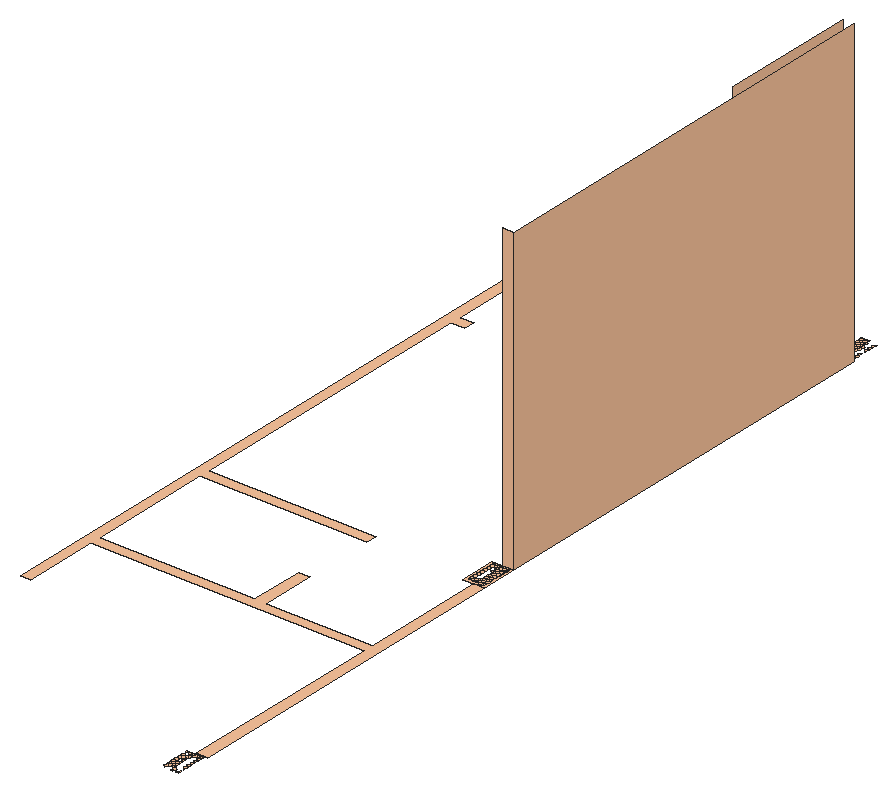
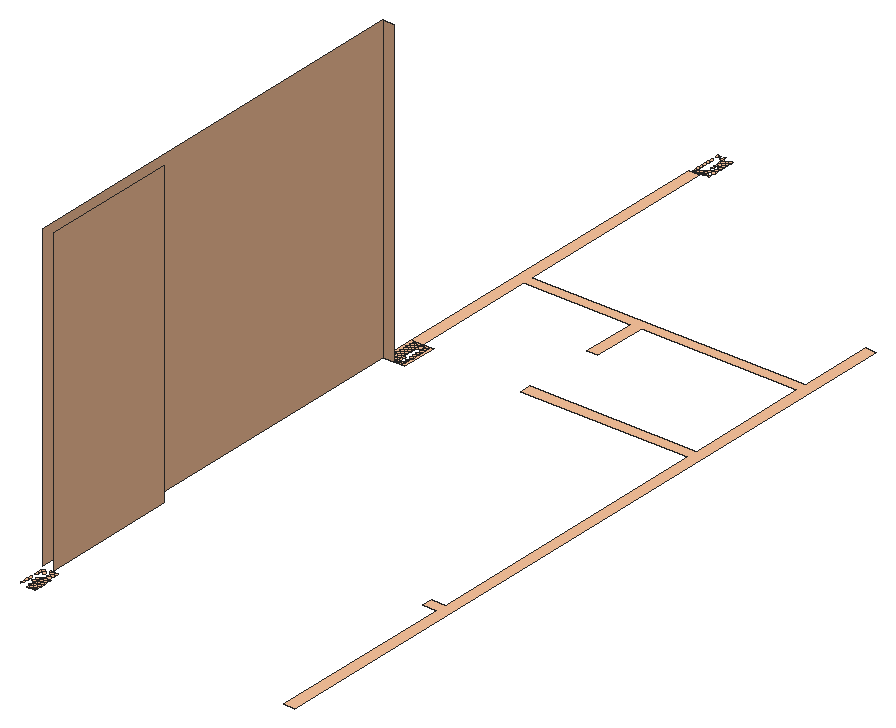
# SketchUp Ruby script. Lengths in inches.
U = 1.inch
M = Sketchup.active_model
def pt(a) = Geom::Point3d.new(a.map { |v| v * U })
def face(e, loops, mat)
  f = e.add_face(loops[0].map { |a| pt(a) })
  loops[1..].each { |l| e.add_face(l.map { |a| pt(a) }).erase! }
  f.material = f.back_material = mat if mat
  f
end
# faces: each face lists its corners as indices into pts; further lists are holes
def faces(e, pts, list, mat = nil) = list.each { |f| face(e, (f[0].is_a?(Array) ? f : [f]).map { |l| l.map { |i| pts[i] } }, mat) }
# xy, xz, yz: faces in a plane at the given z, y or x. An outline is a flat list of corners, or four numbers for a rectangle; further outlines are holes
def ring(l) = l.size == 4 ? [[l[0], l[1]], [l[2], l[1]], [l[2], l[3]], [l[0], l[3]]] : l.each_slice(2).to_a
def flat(e, list, mat, &to3) = list.each { |f| face(e, (f[0].is_a?(Array) ? f : [f]).map { |l| ring(l).map { |u, v| to3.(u, v) } }, mat) }
def xy(e, z, list, mat = nil) = flat(e, list, mat) { |x, y| [x, y, z] }
def xz(e, y, list, mat = nil) = flat(e, list, mat) { |x, z| [x, y, z] }
def yz(e, x, list, mat = nil) = flat(e, list, mat) { |y, z| [x, y, z] }
def lines(e, pts, list) = list.each { |a, b| e.add_line(pt(pts[a]), pt(pts[b])) }
# prism: a flat outline (further loops are holes) pulled along v
def prism(e, loops, v, mat = nil)
  f = face(e, loops, mat); d = Geom::Vector3d.new(v.map { |x| x * U })
  f.pushpull(f.normal.samedirection?(d) ? d.length : -d.length)
end
def box(e, o, s, mat = nil) = prism(e, [[o, [o[0] + s[0], o[1], o[2]], [o[0] + s[0], o[1] + s[1], o[2]], [o[0], o[1] + s[1], o[2]]]], [0, 0, s[2]], mat)
def at(x, y, z, deg = 0) = Geom::Transformation.translation(pt([x, y, z])) * Geom::Transformation.rotation(ORIGIN, Z_AXIS, deg.degrees)
def axes(o, x, y, z) = Geom::Transformation.new([*x, 0, *y, 0, *z, 0, *pt(o).to_a, 1])
def part(name) = M.definitions.add(name)
# library, detail: a bought-in or finely detailed component or shape, given as its bounding box
def library(name, o, s) = part(name).tap { |d| box(d.entities, o, s) }
def detail(e, o, s) = box(e.add_group.entities, o, s)
def put(e, d, t, mat = nil) = e.add_instance(d, t).tap { |i| i.material = mat if mat }
def group(e, t, mat = nil) = e.add_group.tap { |g| g.transformation = t; g.material = mat if mat }.entities
root = M.entities
M.materials.add("[Color A02]1").color = [252, 197, 157]
xy(root,-0.11,[[171.71,213.21,172.47,213.21,172.09,213.59],[173.49,213.21,174.25,213.21,173.87,213.59],[174.25,213.21,174.88,213.21,174.88,214.22,174.69,214.42,173.87,213.59],[168.55,213.59,169.43,214.48,168.55,215.36,167.91,214.73,167.91,214.22],[172.09,213.59,172.98,214.48,172.09,215.36,171.33,214.6,171.33,214.35],
  [171.33,214.35,171.33,214.6,171.21,214.48],[169.43,214.48,170.32,215.36,169.43,216.25,168.55,215.36],[171.21,214.48,171.33,214.6,171.33,216.125,171.21,216.25,170.32,215.36],[167.91,214.73,168.55,215.36,167.91,216],[168.55,215.36,169.43,216.25,168.55,217.14,167.91,216.5,167.91,216],
  [170.32,215.36,171.21,216.25,170.32,217.14,169.43,216.25],[174.88,216,174.88,216.38,174.69,216.1875],[174.69,216.1875,174.88,216.38,174.88,217.77,174.6875,217.96,173.8125,217.08],[169.43,216.25,170.32,217.14,169.43,218.02,168.55,217.14],[171.21,216.25,171.33,216.38,171.33,217.83,171.18,217.99,170.32,217.14],
  [167.91,216.5,168.55,217.14,167.91,217.77],[168.55,217.14,169.43,218.02,168.55,218.91,167.91,218.28,167.91,217.77],[170.32,217.14,171.18,217.99,170.3,218.89,169.43,218.02],[174.88,217.77,174.88,218.15,174.6875,217.96],[174.6875,217.96,174.88,218.15,174.88,219.54,174.6875,219.73,173.8,218.85],
  [171.18,217.99,171.33,218.15,171.33,219.61,171.18,219.77,170.3,218.89],[167.91,218.28,168.55,218.91,167.91,219.54],[168.55,218.91,169.42,219.78,168.54,220.68,167.91,220.05,167.91,219.54],[174.88,219.54,174.88,219.92,174.6875,219.73],[174.6875,219.73,174.88,219.92,174.88,221.32,174.6875,221.51,173.8,220.62],
  [171.18,219.77,171.33,219.92,171.33,221.32,171.14,221.51,170.3,220.66],[167.91,220.05,168.54,220.68,167.91,221.32],[168.54,220.68,169.42,221.56,168.55,222.44,167.91,221.82,167.91,221.32],[174.88,221.32,174.88,221.7,174.6875,221.51],[174.6875,221.51,174.88,221.7,174.88,223.09,174.6875,223.28,173.8,222.39],
  [169.42,221.56,170.26,222.39,169.39,223.26,168.55,222.44],[167.91,221.82,168.55,222.44,167.91,223.09],[170.26,222.39,171.14,223.28,170.29,224.13,169.39,223.26],[168.55,222.44,169.39,223.26,168.5,224.15,167.91,223.6,167.91,223.09],[174.88,223.09,174.88,223.47,174.6875,223.28],
  [171.14,223.28,171.33,223.47,171.33,224.86,171.19,225,170.29,224.13],[174.6875,223.28,174.88,223.47,174.88,224.86,174.6875,225.05,173.8,224.16],[171.33,223.47,172.03,224.16,171.33,224.86],[172.03,224.16,172.92,225.05,172.09,225.88,171.33,225.14,171.33,224.86],[171.33,224.86,171.33,225.14,171.19,225],
  [174.88,224.86,174.88,225.24,174.6875,225.05],[171.19,225,171.33,225.14,171.33,226.13,170.57,226.13,170.3125,225.88],[169.41,225.02,170.3125,225.88,170.07,226.13,168.8,226.13,168.53,225.89],[172.92,225.05,173.8,225.9375,173.61,226.13,172.35,226.13,172.09,225.88],[174.6875,225.05,174.88,225.24,174.88,226.13,173.99,226.13,173.8,225.9375],
  [171.33,225.14,172.09,225.88,171.84,226.13,171.33,226.13],[167.91,225.37,168.53,225.89,168.29,226.13,167.91,226.13],[170.3125,225.88,170.57,226.13,170.07,226.13],[172.09,225.88,172.35,226.13,171.84,226.13],[168.53,225.89,168.8,226.13,168.29,226.13],
  [173.8,225.9375,173.99,226.13,173.61,226.13],[171.33,227.14,171.33,314.26,57.37,314.26,57.37,283.24,52.81,283.24,52.81,585.88,57.37,585.88,57.37,506.23,63.32,506.23,63.32,501.8,57.37,501.8,57.37,375.68,126.89,375.68,126.89,371.24,57.37,371.24,57.37,318.69,122.33,318.69,122.33,341.23,126.89,341.23,126.89,318.69,171.33,318.69,171.33,371.24,175.89,371.24,175.89,227.14],[166.9,371.24,171.33,371.24,171.33,372.26,167.91,372.26,167.91,385.3,171.33,385.3,171.33,386.1875,166.9,386.1875],[171.33,371.24,175.89,371.24,175.89,386.1875,171.33,386.1875,171.33,385.3,174.88,385.3,174.88,372.26,171.33,372.26],[167.91,372.26,168.17,372.26,168.55,372.64,167.91,373.27],
  [168.93,372.26,169.94,372.26,170.32,372.64,169.43,373.52,168.55,372.64],[169.94,372.26,170.7,372.26,170.32,372.64],[170.7,372.26,171.33,372.26,171.33,373.4,171.21,373.52,170.32,372.64],[172.47,372.26,173.49,372.26,173.87,372.64,172.98,373.52,172.09,372.64],[173.49,372.26,174.25,372.26,173.87,372.64],
  [174.25,372.26,174.88,372.26,174.88,373.27,174.69,373.46,173.87,372.64],[168.55,372.64,169.43,373.52,168.55,374.41,167.91,373.78,167.91,373.27],[170.32,372.64,171.21,373.52,170.32,374.41,169.43,373.52],[172.09,372.64,172.98,373.52,172.09,374.41,171.33,373.65,171.33,373.4],[173.87,372.64,174.69,373.46,173.8125,374.36,172.98,373.52],
  [174.88,373.27,174.88,373.65,174.69,373.46],[171.33,373.4,171.33,373.65,171.21,373.52],[174.69,373.46,174.88,373.65,174.88,375.04,174.69,375.23,173.8125,374.36],[171.21,373.52,171.33,373.65,171.33,375.17,171.21,375.3,170.32,374.41],[172.98,373.52,173.8125,374.36,172.93,375.25,172.09,374.41],
  [171.33,373.65,172.09,374.41,171.33,375.17],[167.91,373.78,168.55,374.41,167.91,375.04],[173.8125,374.36,174.69,375.23,173.8125,376.13,172.93,375.25],[168.55,374.41,169.43,375.3,168.55,376.18,167.91,375.55,167.91,375.04],[172.09,374.41,172.93,375.25,172.06,376.14,171.33,375.42,171.33,375.17],
  [174.88,375.04,174.88,375.42,174.69,375.23],[174.69,375.23,174.88,375.42,174.88,376.82,174.69,377.01,173.8125,376.13],[172.93,375.25,173.8125,376.13,172.93,377.02,172.06,376.14],[171.33,375.42,172.06,376.14,171.33,376.88],[167.91,375.55,168.55,376.18,167.91,376.82],
  [173.8125,376.13,174.69,377.01,173.8125,377.9,172.93,377.02],[172.06,376.14,172.93,377.02,172.06,377.92,171.33,377.19,171.33,376.88],[168.55,376.18,169.43,377.07,168.55,377.95,167.91,377.32,167.91,376.82],[172.93,377.02,173.8125,377.9,172.93,378.8,172.06,377.92],[171.33,377.19,172.06,377.92,171.33,378.65],
  [167.91,377.32,168.55,377.95,167.91,378.59],[173.8125,377.9,174.69,378.78,173.8125,379.67,172.93,378.8],[172.06,377.92,172.93,378.8,172.06,379.69,171.33,378.97,171.33,378.65],[168.55,377.95,169.42,378.83,168.53,379.73,167.91,379.09,167.91,378.59],[174.88,378.59,174.88,378.97,174.69,378.78],
  [172.93,378.8,173.8125,379.67,172.93,380.57,172.06,379.69],[171.33,378.97,172.06,379.69,171.33,380.43],[167.91,379.09,168.53,379.73,167.91,380.36],[173.8125,379.67,174.69,380.55,173.82,381.45,172.93,380.57],[172.06,379.69,172.93,380.57,172.06,381.46,171.33,380.74,171.33,380.43],
  [168.53,379.73,169.4,380.62,168.54,381.49,167.91,380.87,167.91,380.36],[174.88,380.36,174.88,380.74,174.69,380.55],[172.93,380.57,173.82,381.45,172.94,382.35,172.06,381.46],[171.18,380.58,171.33,380.74,171.33,382.2,171.15,382.39,170.27,381.5],[171.33,380.74,172.06,381.46,171.33,382.2],
  [167.91,380.87,168.54,381.49,167.91,382.13],[173.82,381.45,174.69,382.33,173.82,383.23,172.94,382.35],[172.06,381.46,172.94,382.35,172.02,383.29,171.33,382.58,171.33,382.2],[168.54,381.49,169.42,382.37,168.54,383.27,167.91,382.64,167.91,382.13],[174.88,382.13,174.88,382.51,174.69,382.33],
  [171.33,382.2,171.33,382.58,171.15,382.39],[174.69,382.33,174.88,382.51,174.88,383.91,174.7,384.11,173.82,383.23],[171.15,382.39,171.33,382.58,171.33,384,171.19,384.14,170.3,383.25],[171.33,382.58,172.02,383.29,171.33,384],[167.91,382.64,168.54,383.27,167.91,383.91],
  [168.54,383.27,169.42,384.15,168.54,385.04,167.91,384.41,167.91,383.91],[172.02,383.29,172.9,384.1875,172.09,385.04,171.33,384.29,171.33,384],[174.88,383.91,174.88,384.29,174.7,384.11],[171.33,384,171.33,384.29,171.19,384.14],[174.7,384.11,174.88,384.29,174.88,385.3,173.99,385.3,173.8,385.1],
  [171.19,384.14,171.33,384.29,171.33,385.3,170.57,385.3,170.32,385.04],[169.42,384.15,170.32,385.04,170.07,385.3,168.8,385.3,168.54,385.04],[172.9,384.1875,173.8,385.1,173.61,385.3,172.35,385.3,172.09,385.04],[171.33,384.29,172.09,385.04,171.84,385.3,171.33,385.3],[167.91,384.41,168.54,385.04,168.29,385.3,167.91,385.3],
  [168.54,385.04,168.8,385.3,168.29,385.3],[170.32,385.04,170.57,385.3,170.07,385.3],[172.09,385.04,172.35,385.3,171.84,385.3],[168.93,564.35,169.94,564.35,170.32,564.73,169.43,565.62,168.55,564.73],[170.7,564.35,171.71,564.35,172.09,564.73,171.21,565.62,170.32,564.73],
  [170.32,564.73,171.21,565.62,170.32,566.5,169.43,565.62],[173.87,564.73,174.69,565.56,173.8125,566.45,172.98,565.62],[174.88,565.36,174.88,565.74,174.69,565.56],[174.69,565.56,174.88,565.74,174.88,567.14,174.6875,567.33,173.8125,566.45],[169.43,565.62,170.32,566.5,169.43,567.39,168.55,566.5],
  [172.98,565.62,173.8125,566.45,172.93,567.34,172.09,566.5],[170.32,566.5,171.21,567.39,170.32,568.28,169.43,567.39],[174.88,567.14,174.88,567.52,174.6875,567.33],[174.6875,567.33,174.88,567.52,174.88,568.91,174.6875,569.1,173.8,568.21],[169.43,567.39,170.32,568.28,169.43,569.16,168.55,568.28],
  [170.32,568.28,171.18,569.13,170.3,570.03,169.43,569.16],[171.18,569.13,171.33,569.29,171.33,570.68,171.14,570.87,170.3,570.03],[169.43,569.16,170.3,570.03,169.42,570.92,168.55,570.05],[171.33,569.29,172.03,569.99,171.33,570.68],[167.91,569.42,168.55,570.05,167.91,570.68],
  [172.03,569.99,172.92,570.87,172.03,571.76,171.33,571.0625,171.33,570.68],[170.3,570.03,171.14,570.87,170.26,571.76,169.42,570.92],[168.55,570.05,169.42,570.92,168.54,571.82,167.91,571.1875,167.91,570.68],[171.33,570.68,171.33,571.0625,171.14,570.87],[174.88,570.68,174.88,571.0625,174.6875,570.87],
  [171.14,570.87,171.33,571.0625,171.33,572.46,171.14,572.65,170.26,571.76],[174.6875,570.87,174.88,571.0625,174.88,572.46,174.6875,572.65,173.8,571.76],[169.42,570.92,170.26,571.76,169.37,572.65,168.54,571.82],[171.33,571.0625,172.03,571.76,171.33,572.46],[167.91,571.1875,168.54,571.82,167.91,572.46],
  [170.26,571.76,171.14,572.65,170.26,573.53,169.37,572.65],[172.03,571.76,172.92,572.65,172.03,573.53,171.33,572.84,171.33,572.46],[168.54,571.82,169.37,572.65,168.49,573.52,167.91,572.96,167.91,572.46],[171.33,572.46,171.33,572.84,171.14,572.65],[174.88,572.46,174.88,572.84,174.6875,572.65],
  [169.37,572.65,170.26,573.53,169.39,574.4,168.49,573.52],[171.14,572.65,171.33,572.84,171.33,574.23,171.14,574.42,170.26,573.53],[174.6875,572.65,174.88,572.84,174.88,574.23,174.6875,574.42,173.8,573.53],[171.33,572.84,172.03,573.53,171.33,574.23],[167.91,572.96,168.49,573.52,167.91,574.1],
  [168.49,573.52,169.39,574.4,168.5,575.29,167.91,574.73,167.91,574.1],[170.26,573.53,171.14,574.42,170.29,575.27,169.39,574.4],[169.39,574.4,170.29,575.27,169.41,576.16,168.5,575.29],[171.14,574.42,171.33,574.61,171.33,576,171.19,576.14,170.29,575.27],[174.6875,574.42,174.88,574.61,174.88,576,174.6875,576.19,173.8,575.3],
  [171.33,574.61,172.03,575.3,171.33,576],[167.91,574.73,168.5,575.29,167.91,575.875],[170.29,575.27,171.19,576.14,170.3125,577.02,169.41,576.16],[168.5,575.29,169.41,576.16,168.53,577.03,167.91,576.51,167.91,575.875],[171.33,576,171.33,576.28,171.19,576.14],
  [174.88,576,174.88,576.38,174.6875,576.19],[171.19,576.14,171.33,576.28,171.33,577.27,170.57,577.27,170.3125,577.02],[169.41,576.16,170.3125,577.02,170.07,577.27,168.8,577.27,168.53,577.03],[167.91,576.51,168.53,577.03,168.29,577.27,167.91,577.27],[170.3125,577.02,170.57,577.27,170.07,577.27],
  [168.53,577.03,168.8,577.27,168.29,577.27]],"[Color A02]1")
xz(root,386.1875,[[171.33,-0.11,175.89,125.89]],"[Color A02]1")
yz(root,171.33,[[506.23,-0.11,563.34,125.89]],"[Color A02]1")
yz(root,175.89,[[386.1875,-0.11,563.34,125.89]],"[Color A02]1")
